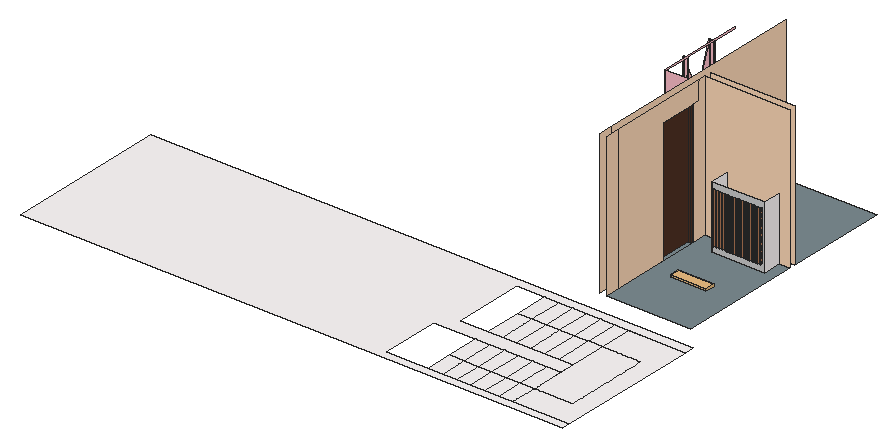
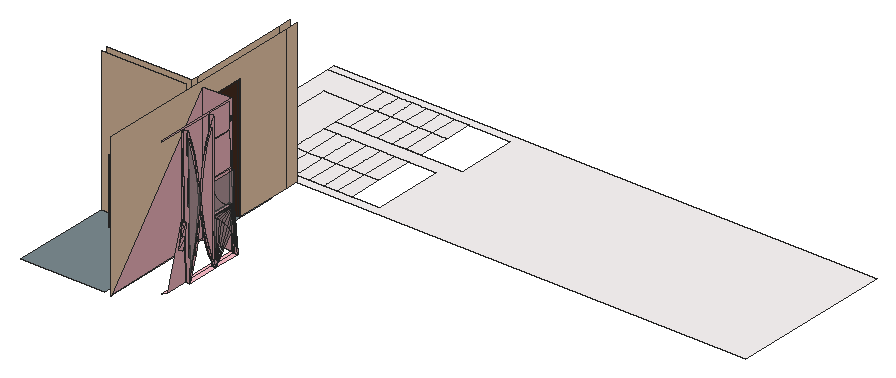
# SketchUp Ruby script. Lengths in inches.
U = 1.inch
M = Sketchup.active_model
def pt(a) = Geom::Point3d.new(a.map { |v| v * U })
def face(e, loops, mat)
  f = e.add_face(loops[0].map { |a| pt(a) })
  loops[1..].each { |l| e.add_face(l.map { |a| pt(a) }).erase! }
  f.material = f.back_material = mat if mat
  f
end
# faces: each face lists its corners as indices into pts; further lists are holes
def faces(e, pts, list, mat = nil) = list.each { |f| face(e, (f[0].is_a?(Array) ? f : [f]).map { |l| l.map { |i| pts[i] } }, mat) }
# xy, xz, yz: faces in a plane at the given z, y or x. An outline is a flat list of corners, or four numbers for a rectangle; further outlines are holes
def ring(l) = l.size == 4 ? [[l[0], l[1]], [l[2], l[1]], [l[2], l[3]], [l[0], l[3]]] : l.each_slice(2).to_a
def flat(e, list, mat, &to3) = list.each { |f| face(e, (f[0].is_a?(Array) ? f : [f]).map { |l| ring(l).map { |u, v| to3.(u, v) } }, mat) }
def xy(e, z, list, mat = nil) = flat(e, list, mat) { |x, y| [x, y, z] }
def xz(e, y, list, mat = nil) = flat(e, list, mat) { |x, z| [x, y, z] }
def yz(e, x, list, mat = nil) = flat(e, list, mat) { |y, z| [x, y, z] }
def lines(e, pts, list) = list.each { |a, b| e.add_line(pt(pts[a]), pt(pts[b])) }
# prism: a flat outline (further loops are holes) pulled along v
def prism(e, loops, v, mat = nil)
  f = face(e, loops, mat); d = Geom::Vector3d.new(v.map { |x| x * U })
  f.pushpull(f.normal.samedirection?(d) ? d.length : -d.length)
end
def box(e, o, s, mat = nil) = prism(e, [[o, [o[0] + s[0], o[1], o[2]], [o[0] + s[0], o[1] + s[1], o[2]], [o[0], o[1] + s[1], o[2]]]], [0, 0, s[2]], mat)
def at(x, y, z, deg = 0) = Geom::Transformation.translation(pt([x, y, z])) * Geom::Transformation.rotation(ORIGIN, Z_AXIS, deg.degrees)
def axes(o, x, y, z) = Geom::Transformation.new([*x, 0, *y, 0, *z, 0, *pt(o).to_a, 1])
def part(name) = M.definitions.add(name)
# library, detail: a bought-in or finely detailed component or shape, given as its bounding box
def library(name, o, s) = part(name).tap { |d| box(d.entities, o, s) }
def detail(e, o, s) = box(e.add_group.entities, o, s)
def put(e, d, t, mat = nil) = e.add_instance(d, t).tap { |i| i.material = mat if mat }
def group(e, t, mat = nil) = e.add_group.tap { |g| g.transformation = t; g.material = mat if mat }.entities
root = M.entities
M.materials.add("Polis06_194").color = [79, 50, 36]
M.materials.add("[0006_Pink]").color = [255, 192, 203]
M.materials.add("[0007_MistyRose]").color = [255, 228, 225]
M.materials.add("[0010_Snow]").color = [255, 250, 250]
M.materials.add("[0027_PeachPuff]").color = [255, 218, 185]
M.materials.add("[Carrera Marble]").color = [207, 207, 207]
M.materials.add("[Concrete Pavers Block Multi]").color = [124, 140, 145]
M.materials.add("[Translucent Glass Gray]").color = [128, 128, 128]
M.materials["[Translucent Glass Gray]"].alpha = 0.5
M.materials.add("[Wood Veneer 02]").color = [190, 128, 91]
c1 = part("Flush door")
xy(c1.entities,0,[[0,0,4.72,1.18],[0,34.25,4.72,35.43]],"Polis06_194")
xy(c1.entities,85.26,[[0,1.18,4.72,34.25]],"Polis06_194")
xy(c1.entities,86.61,[[0,0,4.72,35.43]],"Polis06_194")
xz(c1.entities,0,[[0,0,4.72,86.61]],"Polis06_194")
xz(c1.entities,1.18,[[0,0,2.36,85.26],[2.36,0,4.72,85.26]],"Polis06_194")
xz(c1.entities,34.25,[[0,0,4.72,85.26]],"Polis06_194")
xz(c1.entities,35.43,[[0,0,4.72,86.61]],"Polis06_194")
yz(c1.entities,0,[[0,0,1.18,86.61],[34.25,0,35.43,86.61],[1.18,85.26,34.25,86.61]],"Polis06_194")
yz(c1.entities,2.36,[[1.18,0,34.25,0,34.25,85.21,1.18,85.26]],"Polis06_194")
yz(c1.entities,4.72,[[0,0,1.18,86.61],[34.25,0,35.43,86.61],[1.18,85.26,34.25,86.61]],"Polis06_194")
c2 = library("toilet 2",[0.13,0,0],[30.44,8.22,2])
xy(root,-7.5625,[[109.5625,0,571.5625,0,571.5625,6.25,415.5625,6.25,415.5625,57.9375,523.5625,57.9375,523.5625,70.375,427.5625,70.375,427.5625,130.875,571.5625,130.875,571.5625,138.9375,109.5625,138.9375],[451.5625,6.25,463.5625,29.875],[463.5625,6.25,475.5625,29.875],[475.5625,6.25,487.5625,29.875],[487.5625,6.25,499.5625,29.875],
  [499.5625,6.25,511.5625,29.875],[511.5625,6.25,523.5625,29.875],[523.5625,6.25,571.5625,6.25,571.5625,130.875,523.5625,130.875,523.5625,102.3125,556.33,102.3125,556.33,29.875,523.5625,29.875],[451.5625,29.875,463.5625,57.9375],[463.5625,29.875,475.5625,57.9375],
  [475.5625,29.875,487.5625,57.9375],[487.5625,29.875,499.5625,57.9375],[499.5625,29.875,511.5625,57.9375],[511.5625,29.875,523.5625,57.9375],[523.5625,29.875,556.33,102.3125],
  [451.5625,70.375,463.5625,102.3125],[463.5625,70.375,475.5625,102.3125],[475.5625,70.375,487.5625,102.3125],[487.5625,70.375,499.5625,102.3125],[499.5625,70.375,511.5625,102.3125],
  [511.5625,70.375,523.5625,102.3125],[451.5625,102.3125,463.5625,130.875],[463.5625,102.3125,475.5625,130.875],[475.5625,102.3125,487.5625,130.875],[487.5625,102.3125,499.5625,130.875],
  [499.5625,102.3125,511.5625,130.875],[511.5625,102.3125,523.5625,130.875]],"[0010_Snow]")
xy(root,0,[[508.61,237.66,553.2,252.9375],[500.21,258.9375,543.78,274.78]],"[0010_Snow]")
xy(root,0,[[484.5625,240.51,490.5625,246.2]],"[0027_PeachPuff]")
xy(root,0,[[490.5625,147.9375,562.5625,147.9375,562.5625,252.9375,553.2,252.9375,553.2,237.66,508.61,237.66,508.61,252.9375,490.5625,252.9375],[483.52,177.19,490.5625,240.51],[490.5625,258.9375,500.21,258.9375,500.21,274.78,543.78,274.78,543.78,258.9375,562.5625,258.9375,562.5625,345.21,490.5625,345.21]],"[Concrete Pavers Block Multi]")
xy(root,0.5,[[453.17,250.71,456.54,272.96],[453.17,273.46,456.54,301.21]],"[0006_Pink]")
xy(root,5.99,[[510.4375,236.375,511.58,237.09],[512.87,236.375,514.01,237.09],[515.3,236.375,516.4375,237.09],[517.73,236.375,518.87,237.09],[520.16,236.375,521.3,237.09],
  [522.59,236.375,523.73,237.09],[525.02,236.375,526.16,237.09],[527.45,236.375,528.59,237.09],[529.88,236.375,531.02,237.09],[531.83,236.375,532.97,237.09],
  [534.125,236.375,535.26,237.09],[536.42,236.375,537.55,237.09],[538.71,236.375,539.85,237.09],[541,236.375,542.14,237.09],[543.3,236.375,544.43,237.09],
  [545.59,236.375,546.73,237.09],[547.88,236.375,549.02,237.09],[550.18,236.375,551.3125,237.09],[510.4375,237.09,531.02,237.66],[531.51,237.09,551.3125,237.66]],"[0010_Snow]")
xy(root,6.2,[[502.06,274.78,521.41,275.36],[521.88,274.78,542,275.36],[502.06,275.36,503.17,276.11],[504.3,275.36,505.41,276.11],[506.54,275.36,507.65,276.11],
  [508.78,275.36,509.89,276.11],[511.02,275.36,512.13,276.11],[513.26,275.36,514.37,276.11],[515.5,275.36,516.61,276.11],[517.74,275.36,518.85,276.11],
  [519.98,275.36,521.09,276.11],[521.88,275.36,522.99,276.11],[524.26,275.36,525.37,276.11],[526.63,275.36,527.74,276.11],[529.01,275.36,530.12,276.11],
  [531.38,275.36,532.5,276.11],[533.76,275.36,534.87,276.11],[536.13,275.36,537.25,276.11],[538.51,275.36,539.62,276.11],[540.89,275.36,542,276.11]],"[0010_Snow]")
xy(root,37.375,[[456.0625,250.71,459.4375,272.96]],"[0006_Pink]")
xy(root,37.875,[[456.0625,250.71,459.4375,272.96]],"[0006_Pink]")
xz(root,207.77,[[484.5625,0,490.5625,105.5625]],"[0027_PeachPuff]")
xz(root,236.375,[[510.4375,5.99,511.58,48.56],[512.87,5.99,514.01,48.56],[515.3,5.99,516.4375,48.56],[517.73,5.99,518.87,48.56],[520.16,5.99,521.3,48.56],
  [522.59,5.99,523.73,48.56],[525.02,5.99,526.16,48.56],[527.45,5.99,528.59,48.56],[529.88,5.99,531.02,48.56],[531.83,5.99,532.97,48.56],
  [534.125,5.99,535.26,48.56],[536.42,5.99,537.55,48.56],[538.71,5.99,539.85,48.56],[541,5.99,542.14,48.56],[543.3,5.99,544.43,48.56],
  [545.59,5.99,546.73,48.56],[547.88,5.99,549.02,48.56],[550.18,5.99,551.3125,48.56]],"[Wood Veneer 02]")
xz(root,237.09,[[510.4375,5.99,511.58,48.56],[511.58,5.99,512.87,48.56],[512.87,5.99,514.01,48.56],[514.01,5.99,515.3,48.56],[515.3,5.99,516.4375,48.56],
  [516.4375,5.99,517.73,48.56],[517.73,5.99,518.87,48.56],[518.87,5.99,520.16,48.56],[520.16,5.99,521.3,48.56],[521.3,5.99,522.59,48.56],
  [522.59,5.99,523.73,48.56],[523.73,5.99,525.02,48.56],[525.02,5.99,526.16,48.56],[526.16,5.99,527.45,48.56],[527.45,5.99,528.59,48.56],
  [529.88,5.99,531.02,48.56],[531.51,5.99,531.83,48.56],[531.83,5.99,532.97,48.56],[532.97,5.99,534.125,48.56],[534.125,5.99,535.26,48.56],
  [535.26,5.99,536.42,48.56],[536.42,5.99,537.55,48.56],[537.55,5.99,538.71,48.56],[538.71,5.99,539.85,48.56],[539.85,5.99,541,48.56],
  [541,5.99,542.14,48.56],[542.14,5.99,543.3,48.56],[543.3,5.99,544.43,48.56],[544.43,5.99,545.59,48.56],[545.59,5.99,546.73,48.56],
  [546.73,5.99,547.88,48.56],[547.88,5.99,549.02,48.56],[549.02,5.99,550.18,48.56],[550.18,5.99,551.3125,48.56]],"[0010_Snow]")
xz(root,237.09,[[528.59,5.99,529.88,48.56]],"[Wood Veneer 02]")
xz(root,237.66,[[[508.61,0,553.2,53.66],[510.4375,5.99,531.02,48.56],[531.51,5.99,551.3125,48.56]]],"[Carrera Marble]")
xz(root,240.51,[[484.5625,0,490.5625,105.5625]],"[0027_PeachPuff]")
xz(root,249.21,[[459.4375,0,484.5625,0,484.33,0.5,484.5625,116.8125,459.4375,116.8125]],"[0006_Pink]")
xz(root,250.71,[[453.17,0.5,456.54,0.5,457.47,37.375,456.0625,37.375],[456.54,0.5,459.4375,37.375,457.47,37.375],[457.47,37.375,459.4375,37.375,459.4375,37.875,457.48,37.875],[456.0625,37.875,457.48,37.875,458.13,63.875,456.0625,63.875],[457.48,37.875,459.4375,37.875,459.4375,63.875,458.13,63.875]],"[0006_Pink]")
xz(root,252.9375,[[490.5625,0,562.5625,121.1875]],"[0027_PeachPuff]")
xz(root,252.9375,[[508.61,0,553.2,53.66]],"[Wood Veneer 02]")
xz(root,258.9375,[[490.5625,0,562.5625,121.1875]],"[0027_PeachPuff]")
xz(root,258.9375,[[500.21,0,543.78,55.54]],"[Wood Veneer 02]")
xz(root,272.96,[[453.17,0.5,456.0625,37.375,459.4375,37.375,456.54,0.5],[456.0625,37.875,459.4375,63.875]],"[0006_Pink]")
xz(root,273.46,[[455.3125,0.5,456.54,0.5,459.4375,115.8125,456.0625,115.8125,456.0625,114.75,455.3125,114.75]],"[0006_Pink]")
xz(root,273.86,[[455.3125,2.32,456.0625,112.97]],"[0006_Pink]")
xz(root,274.78,[[[500.21,0,543.78,55.54],[521.88,6.2,542,50.26],[502.06,6.2,521.41,50.26]]],"[0010_Snow]")
xz(root,275.36,[[502.06,6.2,503.17,50.26],[503.17,6.2,504.3,50.26],[504.3,6.2,505.41,50.26],[505.41,6.2,506.54,50.26],[506.54,6.2,507.65,50.26],
  [507.65,6.2,508.78,50.26],[508.78,6.2,509.89,50.26],[509.89,6.2,511.02,50.26],[511.02,6.2,512.13,50.26],[512.13,6.2,513.26,50.26],
  [513.26,6.2,514.37,50.26],[514.37,6.2,515.5,50.26],[515.5,6.2,516.61,50.26],[516.61,6.2,517.74,50.26],[517.74,6.2,518.85,50.26],
  [518.85,6.2,519.98,50.26],[519.98,6.2,521.09,50.26],[521.09,6.2,521.41,50.26],[521.88,6.2,522.99,50.26],[522.99,6.2,524.26,50.26],
  [524.26,6.2,525.37,50.26],[525.37,6.2,526.63,50.26],[526.63,6.2,527.74,50.26],[527.74,6.2,529.01,50.26],[529.01,6.2,530.12,50.26],
  [530.12,6.2,531.38,50.26],[531.38,6.2,532.5,50.26],[532.5,6.2,533.76,50.26],[533.76,6.2,534.87,50.26],[534.87,6.2,536.13,50.26],
  [536.13,6.2,537.25,50.26],[537.25,6.2,538.51,50.26],[538.51,6.2,539.62,50.26],[539.62,6.2,540.89,50.26]],"[0010_Snow]")
xz(root,275.36,[[540.89,6.2,542,50.26]],"[Wood Veneer 02]")
xz(root,276.11,[[502.06,6.2,503.17,50.26],[504.3,6.2,505.41,50.26],[506.54,6.2,507.65,50.26],[508.78,6.2,509.89,50.26],[511.02,6.2,512.13,50.26],
  [513.26,6.2,514.37,50.26],[515.5,6.2,516.61,50.26],[517.74,6.2,518.85,50.26],[519.98,6.2,521.09,50.26],[521.88,6.2,522.99,50.26],
  [524.26,6.2,525.37,50.26],[526.63,6.2,527.74,50.26],[529.01,6.2,530.12,50.26],[531.38,6.2,532.5,50.26],[533.76,6.2,534.87,50.26],
  [536.13,6.2,537.25,50.26],[538.51,6.2,539.62,50.26],[540.89,6.2,542,50.26]],"[Wood Veneer 02]")
xz(root,300.68,[[455.37,3.27,456.06,113.05]],"[0006_Pink]")
xz(root,301.21,[[453.17,0.5,455.375,0.5,455.375,115.8125],[453.17,0.5,455.375,115.8125,456.0625,115.8125],[453.17,0.5,456.0625,115.8125,459.4375,115.8125,456.54,0.5]],"[0006_Pink]")
xz(root,301.65,[[453.1,0.5,456.54,0.5,459.4375,115.8125,456,115.8125]],"[0006_Pink]")
xz(root,301.71,[[456.54,0.5,459.4375,115.8125,459.4375,46.85]],"[0006_Pink]")
yz(root,455.3125,[[[273.46,0.5,273.46,114.75,277.22,106.79,280.75,97.45,283.53,87.87,285.54,78.09,286.77,68.1875,287.21,58.22,286.86,48.24,285.71,38.33,283.79,28.54,281.09,18.93,277.64,9.5625],[273.86,2.32,277.27,9.71,280.71,19.05,283.4,28.63,285.32,38.39,286.46,48.27,286.81,58.22,286.37,68.15,285.15,78.03,283.14,87.77,280.37,97.33,276.85,106.63,273.86,112.97]]],"[0006_Pink]")
yz(root,456.0625,[[273.86,2.32,273.86,112.97,276.85,106.63,280.37,97.33,283.14,87.77,285.15,78.03,286.37,68.15,286.81,58.22,286.46,48.27,285.32,38.39,283.4,28.63,280.71,19.05,277.27,9.71]],"[0006_Pink]")
yz(root,456.0625,[[250.71,37.875,250.71,63.875,272.96,63.875,272.63,60.83,271.97,57.83,270.99,54.93,269.7,52.15,268.11,49.53,266.25,47.1,264.13,44.88,261.79,42.91,259.24,41.2,256.53,39.78,253.67,38.67],[250.71,37.875,253.67,38.67,256.53,39.78,259.24,41.2,261.79,42.91,264.13,44.88,266.25,47.1,268.11,49.53,269.7,52.15,270.99,54.93,271.97,57.83,272.63,60.83,272.96,63.875,272.96,37.875]],"[Translucent Glass Gray]")
yz(root,459.4375,[[249.21,0,249.21,116.8125,323.46,116.8125,323.46,115.8125,273.46,115.8125,272.96,37.375,250.71,37.375,250.71,37.875,272.96,37.875,272.96,63.875,250.71,63.875,250.71,64.375,272.96,64.375,272.96,93.125,250.71,93.125,250.71,93.625,272.96,93.625,272.96,115.8125,250.71,115.8125]],"[0006_Pink]")
yz(root,484.5625,[[147.9375,0,159.9375,121.1875],[159.9375,0,159.9375,121.1875,345.9375,121.1875,345.9375,0,240.51,0,240.51,105.5625,207.77,105.5625,207.77,0]],"[0027_PeachPuff]")
yz(root,490.5625,[[147.9375,0,159.9375,121.1875],[159.9375,0,207.77,0,207.77,105.5625,246.2,105.5625,246.2,121.1875,159.9375,121.1875],[240.51,0,252.9375,0,252.9375,121.1875,246.2,121.1875,246.2,105.5625,240.51,105.5625]],"[0027_PeachPuff]")
yz(root,500.21,[[258.9375,0,274.78,55.54]],"[0010_Snow]")
yz(root,502.06,[[274.78,6.2,275.36,50.26]],"[0010_Snow]")
yz(root,502.06,[[275.36,6.2,276.11,50.26]],"[Wood Veneer 02]")
yz(root,503.17,[[275.36,6.2,276.11,50.26]],"[Wood Veneer 02]")
yz(root,504.3,[[275.36,6.2,276.11,50.26]],"[Wood Veneer 02]")
yz(root,505.41,[[275.36,6.2,276.11,50.26]],"[Wood Veneer 02]")
yz(root,506.54,[[275.36,6.2,276.11,50.26]],"[Wood Veneer 02]")
yz(root,507.65,[[275.36,6.2,276.11,50.26]],"[Wood Veneer 02]")
yz(root,508.61,[[237.66,0,252.9375,53.66]],"[0010_Snow]")
yz(root,508.78,[[275.36,6.2,276.11,50.26]],"[Wood Veneer 02]")
yz(root,509.89,[[275.36,6.2,276.11,50.26]],"[Wood Veneer 02]")
yz(root,510.4375,[[237.09,5.99,237.66,48.56]],"[0010_Snow]")
yz(root,510.4375,[[236.375,5.99,237.09,48.56]],"[Wood Veneer 02]")
yz(root,511.02,[[275.36,6.2,276.11,50.26]],"[Wood Veneer 02]")
yz(root,511.58,[[236.375,5.99,237.09,48.56]],"[Wood Veneer 02]")
yz(root,512.13,[[275.36,6.2,276.11,50.26]],"[Wood Veneer 02]")
yz(root,512.87,[[236.375,5.99,237.09,48.56]],"[Wood Veneer 02]")
yz(root,513.26,[[275.36,6.2,276.11,50.26]],"[Wood Veneer 02]")
yz(root,514.01,[[236.375,5.99,237.09,48.56]],"[Wood Veneer 02]")
yz(root,514.37,[[275.36,6.2,276.11,50.26]],"[Wood Veneer 02]")
yz(root,515.3,[[236.375,5.99,237.09,48.56]],"[Wood Veneer 02]")
yz(root,515.5,[[275.36,6.2,276.11,50.26]],"[Wood Veneer 02]")
yz(root,516.4375,[[236.375,5.99,237.09,48.56]],"[Wood Veneer 02]")
yz(root,516.61,[[275.36,6.2,276.11,50.26]],"[Wood Veneer 02]")
yz(root,517.73,[[236.375,5.99,237.09,48.56]],"[Wood Veneer 02]")
yz(root,517.74,[[275.36,6.2,276.11,50.26]],"[Wood Veneer 02]")
yz(root,518.85,[[275.36,6.2,276.11,50.26]],"[0010_Snow]")
yz(root,518.87,[[236.375,5.99,237.09,48.56]],"[Wood Veneer 02]")
yz(root,519.98,[[275.36,6.2,276.11,50.26]],"[Wood Veneer 02]")
yz(root,520.16,[[236.375,5.99,237.09,48.56]],"[Wood Veneer 02]")
yz(root,521.09,[[275.36,6.2,276.11,50.26]],"[Wood Veneer 02]")
yz(root,521.3,[[236.375,5.99,237.09,48.56]],"[Wood Veneer 02]")
yz(root,521.41,[[274.78,6.2,275.36,50.26]],"[0010_Snow]")
yz(root,521.88,[[274.78,6.2,275.36,50.26]],"[0010_Snow]")
yz(root,521.88,[[275.36,6.2,276.11,50.26]],"[Wood Veneer 02]")
yz(root,522.59,[[236.375,5.99,237.09,48.56]],"[Wood Veneer 02]")
yz(root,522.99,[[275.36,6.2,276.11,50.26]],"[Wood Veneer 02]")
yz(root,523.73,[[236.375,5.99,237.09,48.56]],"[Wood Veneer 02]")
yz(root,524.26,[[275.36,6.2,276.11,50.26]],"[Wood Veneer 02]")
yz(root,525.02,[[236.375,5.99,237.09,48.56]],"[Wood Veneer 02]")
yz(root,525.37,[[275.36,6.2,276.11,50.26]],"[Wood Veneer 02]")
yz(root,526.16,[[236.375,5.99,237.09,48.56]],"[Wood Veneer 02]")
yz(root,526.63,[[275.36,6.2,276.11,50.26]],"[Wood Veneer 02]")
yz(root,527.45,[[236.375,5.99,237.09,48.56]],"[Wood Veneer 02]")
yz(root,527.74,[[275.36,6.2,276.11,50.26]],"[Wood Veneer 02]")
yz(root,528.59,[[236.375,5.99,237.09,48.56]],"[Wood Veneer 02]")
yz(root,529.01,[[275.36,6.2,276.11,50.26]],"[Wood Veneer 02]")
yz(root,529.88,[[236.375,5.99,237.09,48.56]],"[Wood Veneer 02]")
yz(root,530.12,[[275.36,6.2,276.11,50.26]],"[Wood Veneer 02]")
yz(root,531.02,[[237.09,5.99,237.66,48.56]],"[0010_Snow]")
yz(root,531.02,[[236.375,5.99,237.09,48.56]],"[Wood Veneer 02]")
yz(root,531.38,[[275.36,6.2,276.11,50.26]],"[Wood Veneer 02]")
yz(root,531.51,[[237.09,5.99,237.66,48.56]],"[0010_Snow]")
yz(root,531.83,[[236.375,5.99,237.09,48.56]],"[Wood Veneer 02]")
yz(root,532.5,[[275.36,6.2,276.11,50.26]],"[Wood Veneer 02]")
yz(root,532.97,[[236.375,5.99,237.09,48.56]],"[Wood Veneer 02]")
yz(root,533.76,[[275.36,6.2,276.11,50.26]],"[Wood Veneer 02]")
yz(root,534.125,[[236.375,5.99,237.09,48.56]],"[Wood Veneer 02]")
yz(root,534.87,[[275.36,6.2,276.11,50.26]],"[Wood Veneer 02]")
yz(root,535.26,[[236.375,5.99,237.09,48.56]],"[Wood Veneer 02]")
yz(root,536.13,[[275.36,6.2,276.11,50.26]],"[Wood Veneer 02]")
yz(root,536.42,[[236.375,5.99,237.09,48.56]],"[Wood Veneer 02]")
yz(root,537.25,[[275.36,6.2,276.11,50.26]],"[Wood Veneer 02]")
yz(root,537.55,[[236.375,5.99,237.09,48.56]],"[Wood Veneer 02]")
yz(root,538.51,[[275.36,6.2,276.11,50.26]],"[Wood Veneer 02]")
yz(root,538.71,[[236.375,5.99,237.09,48.56]],"[Wood Veneer 02]")
yz(root,539.62,[[275.36,6.2,276.11,50.26]],"[Wood Veneer 02]")
yz(root,539.85,[[236.375,5.99,237.09,48.56]],"[Wood Veneer 02]")
yz(root,540.89,[[275.36,6.2,276.11,50.26]],"[Wood Veneer 02]")
yz(root,541,[[236.375,5.99,237.09,48.56]],"[Wood Veneer 02]")
yz(root,542,[[274.78,6.2,275.36,50.26]],"[0010_Snow]")
yz(root,542,[[275.36,6.2,276.11,50.26]],"[Wood Veneer 02]")
yz(root,542.14,[[236.375,5.99,237.09,48.56]],"[Wood Veneer 02]")
yz(root,543.3,[[236.375,5.99,237.09,48.56]],"[Wood Veneer 02]")
yz(root,543.78,[[258.9375,0,274.78,55.54]],"[0010_Snow]")
yz(root,544.43,[[236.375,5.99,237.09,48.56]],"[Wood Veneer 02]")
yz(root,545.59,[[236.375,5.99,237.09,48.56]],"[Wood Veneer 02]")
yz(root,546.73,[[236.375,5.99,237.09,48.56]],"[Wood Veneer 02]")
yz(root,547.88,[[236.375,5.99,237.09,48.56]],"[Wood Veneer 02]")
yz(root,549.02,[[236.375,5.99,237.09,48.56]],"[Wood Veneer 02]")
yz(root,550.18,[[236.375,5.99,237.09,48.56]],"[Wood Veneer 02]")
yz(root,551.3125,[[237.09,5.99,237.66,48.56]],"[0010_Snow]")
yz(root,551.3125,[[236.375,5.99,237.09,48.56]],"[Wood Veneer 02]")
yz(root,553.2,[[237.66,0,252.9375,53.66]],"[0010_Snow]")
p = [[456.54,301.65,0.5],[456.54,301.71,0.5],[456.54,320.52,0.5],[459.4375,323.46,0],[459.4375,249.21,0],[456.54,250.71,0.5],
  [456.54,272.96,0.5],[456.54,273.46,0.5],[456.54,301.21,0.5],[459.4375,250.71,115.8125],[458.88,250.71,93.625],[458.87,250.71,93.125],
  [458.15,250.71,64.375],[458.13,250.71,63.875],[457.48,250.71,37.875],[457.47,250.71,37.375],[484.5625,249.21,0],[484.5625,345.9375,0],
  [484.33,249.21,0.5],[484.5625,249.21,116.8125],[453.17,250.71,0.5],[456.0625,250.71,37.375],[453.39,251.08,4.22],[454.61,257.28,21.6875],
  [453.17,272.96,0.5],[454.36,255.48,18.42],[454.87,259.33,24.8],[455.11,261.63,27.74],[455.36,264.16,30.49],[455.6,266.91,33.02],
  [455.84,269.84,35.32],[456.0625,272.96,37.375],[459.4375,273.46,115.8125],[459.4375,272.96,37.375],[455.3125,273.46,0.5],[455.3125,277.64,9.5625],
  [453.4,277.64,9.5625],[453.17,273.46,0.5],[456.0625,301.21,115.8125],[453.17,301.21,0.5],[454.63,287.21,58.22],[455.36,297.53,106.63],
  [455.375,301.21,115.8125],[455.375,301.21,0.5],[455.36,297.53,9.68],[455.34,294.5,19.09],[455.33,292.12,28.69],[455.32,290.42,38.44],
  [455.3125,289.39,48.27],[455.3125,289.05,58.16],[455.3125,289.39,68.04],[455.32,290.42,77.88],[455.33,292.12,87.62],[455.34,294.5,97.22],
  [455.33,292.65,28.8],[455.34,295.01,19.24],[455.36,298.04,9.86],[455.37,300.68,3.27],[455.37,300.68,113.05],[455.36,298.04,106.45],
  [455.34,295.01,97.07],[455.33,292.65,87.51],[455.32,290.95,77.8],[455.32,289.92,68],[455.32,289.58,58.16],[455.32,289.92,48.31],
  [455.32,290.95,38.51],[453.38,297.53,9.68],[456.05,298.03,9.86],[456.06,300.68,3.27],[459.4375,301.21,115.8125],[459.4375,301.65,115.8125],
  [459.4375,301.71,115.8125],[459.4375,301.71,46.85],[456.0625,273.86,2.32],[456.0625,277.27,9.71],[455.3125,277.27,9.71],[455.3125,273.86,2.32],
  [456.03,295.01,19.24],[456.02,292.64,28.8],[456.01,290.94,38.51],[456,289.92,48.31],[456,289.58,58.16],[456,289.92,68],
  [456.01,290.94,77.8],[456.02,292.64,87.51],[456.03,295.01,97.07],[456.05,298.03,106.45],[456.06,300.68,113.05],[453.63,251.74,7.89],
  [453.87,252.7,11.5],[455.3125,281.09,18.93],[453.63,281.09,18.93],[456.0625,280.71,19.05],[455.3125,280.71,19.05],[453.6,294.49,19.09],
  [454.11,253.95,15.01],[455.3125,283.79,28.54],[453.88,283.79,28.54],[456.0625,283.4,28.63],[455.3125,283.4,28.63],[453.83,292.12,28.69],
  [453.8,308.31,28.26],[454.05,306.07,38.09],[456,309.18,28.5],[455.3125,285.71,38.33],[454.125,285.72,38.33],[456,306.96,38.25],
  [456.75,306.96,38.25],[456.75,309.18,28.5],[456.0625,285.32,38.39],[455.3125,285.32,38.39],[454.0625,290.41,38.4375],[454.3,304.72,48.08],
  [456,305.625,48.16],[456.75,305.625,48.16],[454.375,286.86,48.24],[455.3125,286.86,48.24],[456.0625,286.46,48.27],[455.3125,286.46,48.27],
  [454.31,289.38,48.27]]
faces(root,p,[[0,1,2,3,4,5,6,7,8],[16,17,18],[19,18,17],[32,7,6],[6,33,32],[34,35,36,37],[[41,42,43,44,45,46,47,48,49,50,51,52,53],[54,55,56,57,58,59,60,61,62,63,64,65,66]],[67,39,68],
  [39,67,44,43],[69,68,39],[39,38,69],[70,71,0,8],[0,1,72,71],[1,2,73],[74,75,76,77],[78,79,80,81,82,83,84,85,86,87,88,69,68],
  [68,69,57,56],[88,69,38],[35,91,92,36],[75,93,94,76],[95,67,78],[67,95,45,44],[68,78,67],[78,68,56,55],
  [91,97,98,92],[93,99,100,94],[101,95,79],[95,101,46,45],[78,79,95],[79,78,55,54],[102,103,104],[97,105,106,98],
  [107,104,103],[108,107,104,109],[99,110,111,100],[101,112,46],[112,101,80],[47,46,112],[79,80,101],[80,79,54,66],
  [103,113,107],[114,107,113],[115,114,107,108],[116,106,117],[105,117,106],[110,118,119,111],[112,120,47],[120,112,81],
  [48,47,120],[80,81,112],[81,80,66,65]],"[0006_Pink]")
faces(root,p,[[9,10,11,12,13,14,15,5,4]],"[0007_MistyRose]")
faces(root,p,[[20,21,22],[23,24,25],[26,24,23],[27,24,26],[28,24,27],[29,24,28],[30,24,29],[31,24,30],
  [38,39,40],[89,22,21],[90,89,21],[96,90,21],[25,96,21],[23,25,21],[26,23,21],[27,26,21],
  [28,27,21],[29,28,21],[30,29,21],[31,30,21]],"[Translucent Glass Gray]")
put(root,c1,axes([484.8,207.77,0],[0.95,0,0],[0,0.912,0],[0,0,1.21877]),"[0006_Pink]")
put(root,c2,at(508.21,193.79,0))
